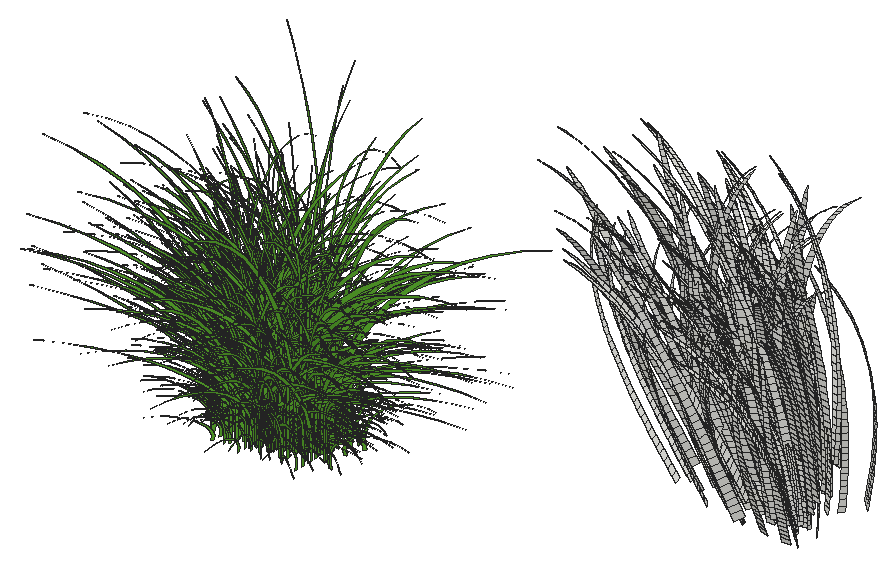
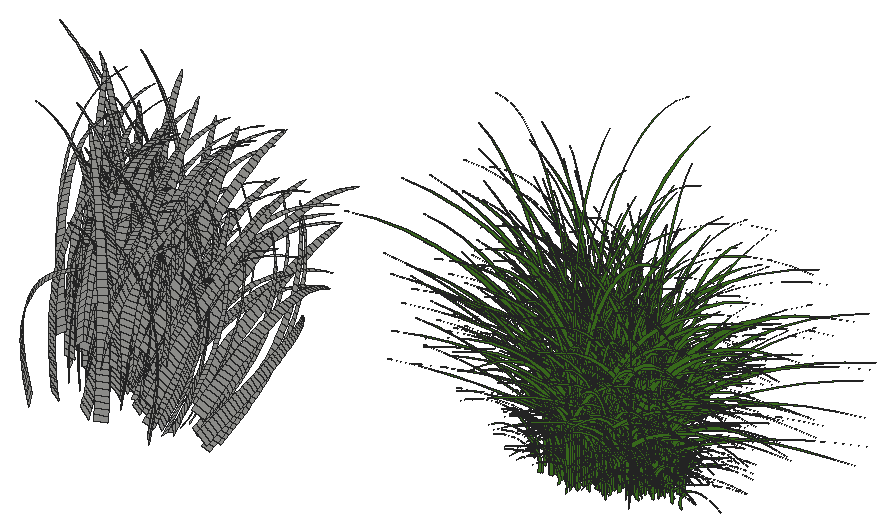
# SketchUp Ruby script. Lengths in inches.
U = 1.inch
M = Sketchup.active_model
def pt(a) = Geom::Point3d.new(a.map { |v| v * U })
def face(e, loops, mat)
  f = e.add_face(loops[0].map { |a| pt(a) })
  loops[1..].each { |l| e.add_face(l.map { |a| pt(a) }).erase! }
  f.material = f.back_material = mat if mat
  f
end
# faces: each face lists its corners as indices into pts; further lists are holes
def faces(e, pts, list, mat = nil) = list.each { |f| face(e, (f[0].is_a?(Array) ? f : [f]).map { |l| l.map { |i| pts[i] } }, mat) }
# xy, xz, yz: faces in a plane at the given z, y or x. An outline is a flat list of corners, or four numbers for a rectangle; further outlines are holes
def ring(l) = l.size == 4 ? [[l[0], l[1]], [l[2], l[1]], [l[2], l[3]], [l[0], l[3]]] : l.each_slice(2).to_a
def flat(e, list, mat, &to3) = list.each { |f| face(e, (f[0].is_a?(Array) ? f : [f]).map { |l| ring(l).map { |u, v| to3.(u, v) } }, mat) }
def xy(e, z, list, mat = nil) = flat(e, list, mat) { |x, y| [x, y, z] }
def xz(e, y, list, mat = nil) = flat(e, list, mat) { |x, z| [x, y, z] }
def yz(e, x, list, mat = nil) = flat(e, list, mat) { |y, z| [x, y, z] }
def lines(e, pts, list) = list.each { |a, b| e.add_line(pt(pts[a]), pt(pts[b])) }
# prism: a flat outline (further loops are holes) pulled along v
def prism(e, loops, v, mat = nil)
  f = face(e, loops, mat); d = Geom::Vector3d.new(v.map { |x| x * U })
  f.pushpull(f.normal.samedirection?(d) ? d.length : -d.length)
end
def box(e, o, s, mat = nil) = prism(e, [[o, [o[0] + s[0], o[1], o[2]], [o[0] + s[0], o[1] + s[1], o[2]], [o[0], o[1] + s[1], o[2]]]], [0, 0, s[2]], mat)
def at(x, y, z, deg = 0) = Geom::Transformation.translation(pt([x, y, z])) * Geom::Transformation.rotation(ORIGIN, Z_AXIS, deg.degrees)
def axes(o, x, y, z) = Geom::Transformation.new([*x, 0, *y, 0, *z, 0, *pt(o).to_a, 1])
def part(name) = M.definitions.add(name)
# library, detail: a bought-in or finely detailed component or shape, given as its bounding box
def library(name, o, s) = part(name).tap { |d| box(d.entities, o, s) }
def detail(e, o, s) = box(e.add_group.entities, o, s)
def put(e, d, t, mat = nil) = e.add_instance(d, t).tap { |i| i.material = mat if mat }
def group(e, t, mat = nil) = e.add_group.tap { |g| g.transformation = t; g.material = mat if mat }.entities
root = M.entities
M.materials.add("[Color_G08]").color = [89, 170, 45]
c1 = part("Miscanthus Gracillimus Blades")
xz(c1.entities,0,[[29.29,0,29.21,4.14,28.62,8.24,27.52,12.24,25.9375,16.07,23.89,19.67,21.41,22.98,18.53,25.97,15.3125,28.57,11.79,30.76,8.03,32.48,4.08,33.73,0,34.48,4.17,33.88,8.22,32.75,12.09,31.1,15.72,28.96,19.03,26.37,21.99,23.37,24.53,20.01,26.61,16.35,28.2,12.45,29.27,8.38,29.8,4.21,29.79,0],[30.59,0,30.59,18.4375,30.42,21.54,29.8,24.59,28.74,27.51,27.27,30.25,25.41,32.74,23.21,34.93,20.7,36.77,17.96,38.23,15.03,39.27,11.98,39.875,8.88,40.02,5.78,39.71,8.9,40.03,12.04,39.89,15.11,39.29,18.07,38.26,20.85,36.81,23.39,34.97,25.64,32.78,27.55,30.29,29.07,27.56,30.19,24.625,30.86,21.5625,31.09,18.4375,31.09,0],[25.43,0,25.6,1.22,25.54,2.45,25.24,3.64,24.72,4.76,24,5.75,23.1,6.59,22.05,7.25,20.9,7.6875,19.69,7.9,18.46,7.875,17.26,7.62,16.125,7.14,17.28,7.63,18.51,7.9,19.77,7.94,21.02,7.74,22.2,7.3125,23.28,6.67,24.23,5.84,25,4.84,25.57,3.72,25.92,2.51,26.04,1.25,25.93,0],[27.07,0,27.07,8.3125,27.03,9.48,26.8,10.63,26.39,11.73,25.8,12.74,25.06,13.64,24.18,14.41,23.18,15.03,22.1,15.48,20.96,15.74,19.79,15.8125,18.63,15.7,17.5,15.39,18.66,15.71,19.85,15.83,21.05,15.77,22.22,15.52,23.34,15.08,24.375,14.47,25.3,13.7,26.09,12.8,26.73,11.78,27.19,10.68,27.48,9.51,27.57,8.3125,27.57,0],[32.33,0,32.33,16.35,32.43,19.17,32.72,21.98,33.19,24.76,33.85,27.5,34.7,30.19,35.73,32.82,36.93,35.37,38.31,37.84,39.84,40.2,41.54,42.46,43.38,44.59,45.37,46.6,43.45,44.56,41.68,42.39,40.04,40.12,38.57,37.74,37.25,35.27,36.09,32.72,35.1,30.1,34.29,27.42,33.66,24.7,33.2,21.93,32.92,19.15,32.83,16.35,32.83,0],
  [33.58,0,33.5625,4.21,34.1,8.38,35.17,12.45,36.76,16.35,38.84,20.01,41.375,23.37,44.33,26.37,47.65,28.96,51.27,31.1,55.14,32.75,59.2,33.88,63.36,34.48,59.29,33.73,55.34,32.48,51.57,30.76,48.05,28.57,44.83,25.97,41.96,22.98,39.48,19.67,37.43,16.07,35.84,12.24,34.75,8.24,34.15,4.14,34.08,0],[36.0625,0,36.0625,8.3125,36.16,9.51,36.44,10.68,36.91,11.78,37.54,12.8,38.34,13.7,39.26,14.47,40.29,15.08,41.41,15.52,42.58,15.77,43.78,15.83,44.98,15.71,46.13,15.39,45,15.7,43.84,15.8125,42.67,15.74,41.53,15.48,40.45,15.03,39.45,14.41,38.57,13.64,37.83,12.74,37.24,11.73,36.83,10.63,36.6,9.48,36.5625,8.3125,36.5625,0],[38.05,0,37.9375,1.25,38.06,2.51,38.41,3.72,38.98,4.84,39.75,5.84,40.7,6.67,41.78,7.3125,42.97,7.74,44.21,7.94,45.47,7.9,46.7,7.63,47.86,7.14,46.72,7.62,45.52,7.875,44.29,7.9,43.08,7.6875,41.93,7.25,40.88,6.59,39.98,5.75,39.26,4.76,38.74,3.64,38.44,2.45,38.38,1.22,38.55,0]],"[Color_G08]")
c2 = part("Grass blade cluster \#1")
put(c2.entities,c1,axes([15.51,50.54,0],[0.60321,-0.79758,0],[0.79758,0.60321,0],[0,0,0.83]))
put(c2.entities,c1,at(0,25.27,0))
c3 = part("Grass blade cluster")
put(c3.entities,c2,axes([30.74,66.43,0],[-0.57215,-0.82015,0],[0.82015,-0.57215,0],[0,0,0.65]))
put(c3.entities,c2,at(0.28,0.71,0))
c4 = part("Grass tuft \#1")
put(c4.entities,c3,at(0,0,0))
put(c4.entities,c3,axes([1.91,58.875,0],[0.17537,-0.9845,0],[0.9845,0.17537,0],[0,0,0.84]))
c5 = part("Grass tuft")
put(c5.entities,c4,at(-0.89,7.45,0))
put(c5.entities,c4,axes([-12.2,31.71,0],[0.80178,-0.59763,0],[0.59763,0.80178,0],[0,0,1.31]))
c6 = part("Ornamental grass clump \#1")
put(c6.entities,c5,axes([-5.64,62.125,0],[0.1788,-0.98389,0],[0.98389,0.1788,0],[0,0,1.27]))
put(c6.entities,c5,at(6.7,0,0))
c7 = part("Ornamental grass clump")
put(c7.entities,c6,at(12.67,21.7,0))
put(c7.entities,c6,axes([-14.56,78.18,0],[0.66352,-1.26381,0],[1.25239,0.65752,0],[0,0,0.9558]))
c8 = part("Miscanthus Gracillimus")
put(c8.entities,c7,axes([-6.55,172.36,0],[-0.09268,-1.60733,0],[1.41765,-0.08174,0],[0,0,1.1742]))
put(c8.entities,c7,at(11.73,20.84,0))
c9 = part("Misc Gracillimus")
put(c9.entities,c8,at(-70.11,-74.01,2.38))
c10 = part("fur_instance\#8")
p = [[-0.25,1.49,0.03],[0.25,-1.49,-0.03],[0.44,-1.47,1.51],[-0.05,1.47,1.57],[0.65,-1.44,3.05],[0.16,1.45,3.11],
  [0.86,-1.42,4.59],[0.38,1.44,4.65],[1.1,-1.39,6.13],[0.62,1.43,6.18],[1.34,-1.35,7.66],[0.875,1.42,7.72],
  [1.6,-1.32,9.19],[1.14,1.41,9.25],[1.88,-1.28,10.72],[1.43,1.41,10.78],[2.18,-1.24,12.25],[1.73,1.41,12.3],
  [2.49,-1.19,13.77],[2.05,1.41,13.82],[2.83,-1.15,15.29],[2.4,1.41,15.34],[3.18,-1.09,16.8],[2.76,1.42,16.85],
  [3.56,-1.03,18.31],[3.14,1.43,18.35],[3.96,-0.97,19.81],[3.55,1.44,19.85],[4.38,-0.91,21.3],[3.99,1.46,21.35],
  [4.84,-0.83,22.78],[4.45,1.48,22.83],[5.32,-0.76,24.26],[4.93,1.51,24.31],[5.82,-0.67,25.73],[5.45,1.54,25.77],
  [6.36,-0.59,27.18],[6,1.57,27.23],[6.93,-0.49,28.625],[6.58,1.61,28.67],[7.54,-0.39,30.05],[7.19,1.66,30.1],
  [8.18,-0.28,31.47],[7.84,1.71,31.51],[8.85,-0.16,32.86],[8.53,1.77,32.9],[9.57,-0.04,34.24],[9.25,1.83,34.27],
  [10.32,0.09,35.59],[10.02,1.9,35.625],[11.12,0.23,36.92],[10.82,1.97,36.95],[11.95,0.38,38.22],[11.67,2.06,38.25],
  [12.84,0.54,39.49],[12.57,2.14,39.52],[13.76,0.71,40.73],[13.51,2.24,40.76],[14.73,0.89,41.93],[14.49,2.34,41.95],
  [15.75,1.08,43.09],[15.52,2.45,43.11],[16.82,1.28,44.2],[16.6,2.5625,44.23],[17.93,1.5,45.27],[17.73,2.68,45.29],
  [19.08,1.73,46.28],[18.9,2.81,46.3],[20.29,1.97,47.24],[20.125,2.93,47.26],[21.53,2.22,48.13],[21.39,3.0625,48.15],
  [22.82,2.5,48.96],[22.7,3.1875,48.98],[24.14,2.8125,49.72],[24.06,3.3,49.73],[25.48,3.27,50.41]]
faces(c10.entities,p,[[0,1,2,3],[3,2,4,5],[5,4,6,7],[7,6,8,9],[9,8,10,11],[11,10,12,13],[13,12,14,15],[15,14,16,17],
  [17,16,18,19],[19,18,20,21],[21,20,22,23],[23,22,24,25],[25,24,26,27],[27,26,28,29],[29,28,30,31],[31,30,32,33],
  [33,32,34,35],[35,34,36,37],[37,36,38,39],[39,38,40,41],[41,40,42,43],[43,42,44,45],[45,44,46,47],[47,46,48,49],
  [49,48,50,51],[51,50,52,53],[53,52,54,55],[55,54,56,57],[57,56,58,59],[59,58,60,61],[61,60,62,63],[63,62,64,65],
  [65,64,66,67],[67,66,68,69],[69,68,70,71],[71,70,72,73],[73,72,74,75],[75,74,76]])
put(root,c9,axes([127.3,24.12,14.73],[0.40613,0,0],[0,0.23,0],[0,0,0.45908]))
put(root,c10,axes([161.89,46.04,18.83],[-0.11569,0.14649,-0.11362],[-0.49612,-0.01353,-0.24569],[-0.28238,-0.00989,0.50725]))
put(root,c10,axes([161.84,45.54,15.92],[0.13882,0.1225,0.02997],[-0.38832,0.05902,-0.33485],[-0.34424,0.00121,0.41007]))
put(root,c10,axes([164.85,44.78,21.47],[-0.38731,-0.08952,-0.1497],[0.42326,-0.11791,0.09629],[-0.18899,-0.03826,0.56909]))
put(root,c10,axes([167.375,46.33,21.8],[-0.5712,-0.00621,-0.12571],[0.08241,-0.15116,0.10787],[-0.15761,-0.00674,0.56684]))
put(root,c10,axes([161.46,45.36,14.86],[0.25376,-0.11142,0.26435],[0.3129,0.07232,0.1949],[-0.33629,0.00118,0.40061]))
put(root,c10,axes([164.68,43.97,18.74],[-0.09562,-0.12227,-0.11226],[0.47205,-0.05859,0.23599],[-0.27058,-0.03426,0.47864]))
put(root,c10,axes([161.26,43.68,14.85],[0.37582,-0.08407,0.27007],[0.14827,0.09994,0.19932],[-0.3433,-0.03091,0.40153]))
put(root,c10,axes([167.84,43.74,19.98],[-0.45134,-0.04336,-0.16335],[0.26487,-0.12485,0.01208],[-0.16324,-0.04231,0.51575]))
put(root,c10,axes([166.53,47.59,18.875],[-0.27902,-0.12125,0.0786],[0.46466,-0.07901,0.25002],[-0.20176,0.02209,0.50718]))
put(root,c10,axes([169.09,42.55,17.125],[-0.34603,0.08867,-0.06121],[-0.25159,-0.06276,-0.21848],[-0.20018,-0.04995,0.40733]))
put(root,c10,axes([163.27,43.46,15.76],[0.37143,-0.07872,0.26996],[0.13229,0.10024,0.18556],[-0.33504,-0.03016,0.39186]))
put(root,c10,axes([164.23,43.5,14.97],[0.28927,0.04096,0.28152],[-0.23066,0.11236,-0.1234],[-0.31438,-0.0283,0.3677]))
put(root,c10,axes([170.18,42.21,17.68],[-0.42495,0.07188,-0.0749],[-0.17281,-0.08134,-0.22626],[-0.18095,-0.06165,0.42446]))
put(root,c10,axes([170.17,44.48,19],[-0.46693,0.04407,-0.14017],[-0.11268,-0.11869,0.01707],[-0.14651,-0.01142,0.47518]))
put(root,c10,axes([169.15,43.8125,16.33],[-0.24594,-0.08141,-0.04983],[0.3096,-0.07753,0.19842],[-0.20231,0.00171,0.38778]))
put(root,c10,axes([169.08,45.1,22.68],[-0.21709,-0.12668,-0.07521],[0.52524,-0.07803,0.15682],[-0.18992,-0.02954,0.56536]))
put(root,c10,axes([171.66,41.45,17.58],[-0.54111,0.06042,0.07587],[-0.19981,-0.07219,-0.37016],[-0.0944,-0.11415,0.43604]))
put(root,c10,axes([165.41,44.12,15.41],[0.35881,-0.03428,0.29675],[0.0665,0.11534,-0.02105],[-0.30461,0.00107,0.36287]))
put(root,c10,axes([171.71,43.03,20.65],[-0.51581,-0.0175,-0.13293],[0.18056,-0.12516,-0.10858],[-0.10807,-0.06258,0.52244]))
put(root,c10,axes([169.72,42.74,18.6],[-0.0707,0.11438,0.11912],[-0.45161,0.01974,-0.21113],[-0.21388,-0.05337,0.43522]))
put(root,c10,axes([167.97,46.0625,15.54],[0.03855,-0.11777,0.25787],[0.43699,0.01768,0.16073],[-0.22604,0.03772,0.38076]))
put(root,c10,axes([170.29,42.21,17.16],[-0.17604,0.10245,0.09767],[-0.39708,-0.00819,-0.20343],[-0.17133,-0.05837,0.40189]))
put(root,c10,axes([171.36,45.2,23.02],[-0.45394,0.1084,-0.0434],[-0.38463,-0.10138,-0.03875],[-0.07351,-0.03167,0.58893]))
put(root,c10,axes([171.03,43.33,17.5],[-0.33805,-0.05461,-0.08887],[0.25639,-0.0976,0.0914],[-0.13824,-0.01588,0.42164]))
put(root,c10,axes([171.04,42.7,17.68],[-0.30117,0.09238,-0.04137],[-0.31304,-0.05917,-0.12952],[-0.1355,-0.03512,0.42811]))
put(root,c10,axes([168.51,44.0625,21.67],[-0.03124,0.13752,0.09977],[-0.56507,0.02087,-0.1473],[-0.1601,-0.0531,0.55264]))
put(root,c10,axes([171.375,45.45,22.85],[-0.45617,0.10631,-0.04963],[-0.37724,-0.10346,-0.0161],[-0.06368,-0.02656,0.58538]))
put(root,c10,axes([170.98,40.94,15.21],[-0.3561,0.08998,0.2615],[-0.45823,-0.02957,-0.27591],[-0.09498,-0.11484,0.43869]))
put(root,c10,axes([171.01,44.45,21.5625],[-0.4634,-0.06206,-0.05309],[0.30711,-0.12341,0.02068],[-0.07005,-0.0322,0.55017]))
put(root,c10,axes([172.18,44.375,22.7],[-0.5539,-0.03134,-0.06208],[0.19807,-0.14029,-0.02574],[-0.06505,-0.0422,0.58034]))
put(root,c10,axes([166.72,44.78,18.39],[0.29385,0.08784,0.11548],[-0.34758,0.09777,-0.2125],[-0.25229,-0.00884,0.4532]))
put(root,c10,axes([166.67,44.3,14.51],[0.29692,-0.06479,0.27774],[0.20048,0.09221,0.0267],[-0.26969,0.01357,0.34365]))
put(root,c10,axes([165.39,45.5,15.54],[0.41573,0.01969,0.20437],[-0.05133,0.12132,-0.2303],[-0.26854,0.02752,0.38268]))
put(root,c10,axes([169.29,44.83,18.13],[0.01538,0.12452,-0.12889],[-0.45208,0.01116,-0.18619],[-0.2031,0.01115,0.43393]))
put(root,c10,axes([166.09,42.1,14.68],[0.4031,-0.04126,0.25346],[-0.04162,0.10161,0.18282],[-0.27306,-0.05722,0.36744]))
put(root,c10,axes([166.92,45.77,15.81],[0.34512,0.07258,0.07648],[-0.23439,0.09857,-0.29696],[-0.26745,0.02741,0.38113]))
put(root,c10,axes([170.17,43.64,14.86],[-0.04139,-0.09921,0.1408],[0.33679,-0.00837,0.20587],[-0.21754,0.02229,0.31]))
put(root,c10,axes([171.3125,41.54,17.35],[-0.27848,0.1037,0.16149],[-0.44453,-0.029,-0.20606],[-0.11622,-0.08309,0.46124]))
put(root,c10,axes([166.42,45.57,14.84],[0.36852,-0.04563,0.28569],[0.16966,0.10995,-0.08547],[-0.26008,0.02666,0.37063]))
put(root,c10,axes([171.5,43.61,14.88],[-0.20225,-0.07964,0.07154],[0.28157,-0.05014,0.22923],[-0.17863,0.02981,0.3009]))
put(root,c10,axes([173.4,44.29,22.76],[-0.55642,0.06257,-0.01207],[-0.1944,-0.1278,-0.0692],[-0.04939,-0.04658,0.57961]))
put(root,c10,axes([168.125,42.74,14.57],[0.31297,-0.02783,0.26111],[0.01775,0.10078,0.01553],[-0.27274,-0.01149,0.31594]))
put(root,c10,axes([172.91,43.47,16.54],[-0.31878,-0.05388,-0.02498],[0.21365,-0.08716,0.18387],[-0.14285,0.01564,0.3591]))
put(root,c10,axes([173.13,49.42,16.5],[-0.47347,-0.07401,0.17022],[0.33824,-0.11173,0.31464],[-0.07498,0.064,0.45544]))
put(root,c10,axes([172.2,43.33,21.07],[-0.25642,0.12058,0.08666],[-0.4804,-0.03631,-0.14745],[-0.10769,-0.06235,0.52058]))
put(root,c10,axes([169.71,42.33,15.98],[0.06935,-0.10181,-0.05617],[0.37358,-0.01131,0.19685],[-0.19972,-0.03626,0.371]))
put(root,c10,axes([168.31,43.01,16.91],[0.28717,0.05906,0.18907],[-0.28878,0.09826,-0.11438],[-0.2288,-0.02897,0.40472]))
put(root,c10,axes([173.67,42.95,17.48],[-0.35379,-0.03909,-0.07768],[0.19159,-0.09858,0.08919],[-0.12272,-0.00957,0.39802]))
put(root,c10,axes([173.29,42.43,16.625],[-0.28182,0.07508,-0.08197],[-0.24497,-0.06261,-0.07961],[-0.12478,-0.01941,0.37146]))
put(root,c10,axes([169.82,43.23,17.05],[0.24853,0.07082,0.13756],[-0.2987,0.08669,-0.15855],[-0.22219,-0.01756,0.38881]))
put(root,c10,axes([171.39,46.29,21.64],[-0.09016,0.14644,-0.14213],[-0.56355,-0.01096,-0.06546],[-0.10497,0.00344,0.55103]))
put(root,c10,axes([173.06,41.56,16.45],[-0.17655,0.0893,0.11813],[-0.36927,-0.01088,-0.17139],[-0.12725,-0.06066,0.36837]))
put(root,c10,axes([166.32,47.12,18.26],[0.49159,0.04485,0.09037],[-0.18613,0.133,-0.23756],[-0.19567,0.02142,0.49187]))
put(root,c10,axes([174.73,41.97,19.27],[-0.54515,0.00019,-0.04346],[0.08112,-0.10399,-0.26579],[-0.02004,-0.09315,0.47314]))
put(root,c10,axes([173.63,43.34,20.02],[-0.38338,-0.06825,-0.0577],[0.32906,-0.10289,-0.00157],[-0.05587,-0.03625,0.49844]))
put(root,c10,axes([166.3125,48.24,15.5],[0.51684,0.0215,0.1164],[-0.05837,0.1295,-0.32132],[-0.20042,0.05174,0.43122]))
put(root,c10,axes([174.5625,42.51,18.33],[-0.42742,0.04491,-0.01878],[-0.13382,-0.09906,-0.04894],[-0.04414,-0.0339,0.44116]))
put(root,c10,axes([174,45.72,20.46],[-0.3694,0.10768,-0.12097],[-0.39548,-0.08499,0.0781],[-0.04054,0.00726,0.51598]))
put(root,c10,axes([171.56,45.57,21.32],[-0.06999,-0.1388,0.09222],[0.54267,-0.03086,0.12251],[-0.12696,-0.00089,0.53285]))
put(root,c10,axes([170.37,42.1,17.375],[0.20583,0.07337,0.22786],[-0.40086,0.07736,-0.05373],[-0.17774,-0.06055,0.41693]))
put(root,c10,axes([174.82,44.43,21.88],[-0.44292,-0.07247,-0.01487],[0.33674,-0.11929,0.04408],[-0.05271,-0.02311,0.54972]))
put(root,c10,axes([172.51,43.86,17.97],[-0.1635,-0.10272,0.04784],[0.41176,-0.05199,0.11457],[-0.1028,-0.00072,0.43144]))
put(root,c10,axes([171.69,42.21,19.13],[-0.00018,0.10449,0.24912],[-0.53072,0.0308,-0.09002],[-0.11758,-0.08407,0.46666]))
put(root,c10,axes([175.04,43.02,17.35],[-0.378,-0.02814,-0.02544],[0.14155,-0.09997,0.10771],[-0.07424,0.00243,0.38971]))
put(root,c10,axes([173.23,43.25,16.97],[-0.18086,-0.08793,0.01093],[0.35575,-0.05669,0.11402],[-0.10899,-0.00466,0.39198]))
put(root,c10,axes([168.98,42.29,16.65],[0.36206,-0.08311,0.07727],[0.22303,0.06894,0.21187],[-0.19897,-0.04965,0.40487]))
put(root,c10,axes([175.14,46.77,16.36],[-0.50255,-0.00379,0.04989],[0.06422,-0.11586,0.30455],[-0.00175,0.05488,0.39355]))
put(root,c10,axes([171.48,41.82,17.45],[0.11839,0.08702,0.23179],[-0.45761,0.05675,-0.0637],[-0.14695,-0.07005,0.4254]))
put(root,c10,axes([174.02,45.53,22.4],[-0.30008,0.13108,-0.04422],[-0.4957,-0.06287,0.00183],[-0.03589,-0.02154,0.57138]))
put(root,c10,axes([175.21,43.53,18.26],[-0.43075,0.03793,-0.02322],[-0.10996,-0.10489,0.02478],[-0.02753,-0.01653,0.43837]))
put(root,c10,axes([172.71,43.81,20.7],[-0.12159,0.12941,0.00902],[-0.51234,-0.01443,-0.05556],[-0.06562,-0.03301,0.52078]))
put(root,c10,axes([172.93,42.79,19.19],[-0.10684,-0.10313,-0.13113],[0.46435,-0.04764,0.07264],[-0.11632,-0.0501,0.46037]))
put(root,c10,axes([171.8125,42.74,18.23],[0.03094,-0.11145,-0.05259],[0.44379,-0.01421,0.12893],[-0.13876,-0.03596,0.43843]))
put(root,c10,axes([170.77,41.62,14.42],[0.30819,-0.01996,0.21867],[-0.08034,0.08385,0.11184],[-0.2146,-0.04497,0.28878]))
put(root,c10,axes([174.24,41.73,17.72],[-0.33936,-0.05842,-0.11874],[0.32052,-0.08468,-0.0844],[-0.04225,-0.05911,0.43914]))
put(root,c10,axes([166.82,44.84,21.55],[0.55538,-0.04347,0.16105],[0.07,0.13775,0.06498],[-0.1844,-0.03733,0.55525]))
put(root,c10,axes([175.91,42.67,20.23],[-0.51823,-0.01807,-0.01549],[0.12857,-0.11474,-0.16499],[0.01257,-0.06919,0.5005]))
put(root,c10,axes([176.18,46.5,21.87],[-0.53194,0.07351,-0.03034],[-0.24436,-0.12866,0.15206],[0.02284,0.00582,0.55711]))
put(root,c10,axes([173.2,43.58,19.65],[-0.10827,0.12148,-0.00042],[-0.4794,-0.01253,-0.05037],[-0.06193,-0.02846,0.48638]))
put(root,c10,axes([176.08,45.47,17.01],[-0.47413,0.01058,0.00606],[-0.00201,-0.1159,0.21118],[-0.00511,0.02935,0.41767]))
put(root,c10,axes([175.33,45.54,22.07],[-0.35953,0.11919,-0.03229],[-0.44475,-0.07957,0.02653],[-0.0137,-0.02083,0.56315]))
put(root,c10,axes([167.76,43.45,21.03],[0.48701,0.04757,0.174],[-0.30593,0.1286,0.04964],[-0.14041,-0.06048,0.55568]))
put(root,c10,axes([168.58,44.0625,19.04],[0.45655,0.02353,0.14229],[-0.16482,0.12487,-0.04265],[-0.1622,-0.02523,0.48286]))
put(root,c10,axes([171.72,43.33,15.77],[0.19405,-0.08782,0.16981],[0.30748,0.04885,0.06553],[-0.16325,0.00896,0.34879]))
put(root,c10,axes([168.82,46.38,18.31],[0.49985,0.00301,0.14964],[-0.02964,0.13367,-0.19035],[-0.18639,0.02041,0.46856]))
put(root,c10,axes([170.82,41.34,14.85],[0.32877,0.00795,0.24484],[-0.22697,0.08276,0.1343],[-0.16825,-0.07161,0.32423]))
put(root,c10,axes([175.875,41.83,16.48],[-0.33843,0.04553,-0.01108],[-0.1473,-0.07721,-0.04176],[-0.03638,-0.02793,0.36355]))
put(root,c10,axes([176.27,44.27,18.79],[-0.41033,0.06923,-0.06032],[-0.23945,-0.09817,0.11027],[-0.00841,0.00619,0.45189]))
put(root,c10,axes([174.74,41.87,16.42],[-0.0905,0.08851,0.04381],[-0.349,-0.00424,-0.10453],[-0.10199,-0.03383,0.35208]))
put(root,c10,axes([175.46,42.67,18.45],[-0.3213,-0.06561,-0.05115],[0.31218,-0.08598,-0.01531],[-0.03754,-0.0354,0.44054]))
put(root,c10,axes([172.41,44.84,19.38],[0.08835,0.12369,-0.09809],[-0.4898,0.03322,-0.09487],[-0.09155,0.003,0.48054]))
put(root,c10,axes([176.61,42.4,18.56],[-0.43764,0.04296,0.02293],[-0.13889,-0.10078,-0.05047],[-0.0046,-0.03883,0.44986]))
put(root,c10,axes([174.37,43.59,21.06],[-0.16558,0.12699,0.05128],[-0.5131,-0.0254,-0.04],[-0.03606,-0.04403,0.52943]))
put(root,c10,axes([174.625,42.89,18.2],[-0.21313,-0.08851,-0.02181],[0.38204,-0.06383,0.0368],[-0.05405,-0.02329,0.43302]))
put(root,c10,axes([172.74,42.17,15.75],[0.21366,-0.07915,0.11274],[0.23837,0.04733,0.13112],[-0.18304,-0.01446,0.32031]))
put(root,c10,axes([175.76,43.25,15.53],[-0.30076,-0.04712,0.07311],[0.21058,-0.07732,0.14762],[-0.03812,0.02306,0.32501]))
put(root,c10,axes([170.98,49.66,16.41],[0.13416,-0.13299,0.35981],[0.57303,0.02622,-0.03812],[-0.07584,0.06473,0.46065]))
put(root,c10,axes([171.11,41.375,15.08],[0.36016,-0.00742,0.21279],[-0.15994,0.08168,0.17492],[-0.16596,-0.07064,0.31982]))
put(root,c10,axes([174.58,42.38,16.63],[0.00161,0.09513,-0.03701],[-0.36368,0.01178,-0.1003],[-0.11093,-0.00865,0.35978]))
put(root,c10,axes([169.46,44.52,19.93],[0.49874,-0.00013,0.14505],[-0.06914,0.13272,-0.04302],[-0.16406,-0.01885,0.50038]))
put(root,c10,axes([174.38,44.55,17.86],[-0.13345,-0.10841,0.09578],[0.43742,-0.04305,0.07746],[-0.05987,0.00506,0.43831]))
put(root,c10,axes([176.63,42.12,18.27],[-0.43123,-0.02453,-0.02633],[0.15077,-0.0963,-0.13931],[0.01076,-0.0592,0.42821]))
put(root,c10,axes([176.64,41.89,16.83],[-0.36718,0.0373,0.01282],[-0.1193,-0.08429,-0.04508],[-0.0113,-0.03262,0.37838]))
put(root,c10,axes([177.61,40.99,16.42],[-0.58089,-0.00691,0.01192],[0.06233,-0.08859,-0.37865],[0.05076,-0.11892,0.43771]))
put(root,c10,axes([176.03,42.23,17.85],[-0.25951,0.08816,0.03471],[-0.34222,-0.05282,-0.03889],[-0.02082,-0.03587,0.42124]))
put(root,c10,axes([174.29,42.03,19.67],[-0.09978,0.10955,0.27884],[-0.57213,-0.00253,-0.05277],[-0.02112,-0.09816,0.49856]))
put(root,c10,axes([174.36,44.22,20.4],[-0.05866,0.12941,-0.03315],[-0.51241,-0.00175,-0.02422],[-0.04091,-0.02008,0.50906]))
put(root,c10,axes([173.59,42.7,16.875],[0.16807,0.08479,0.01084],[-0.34402,0.05473,-0.11203],[-0.11678,-0.00911,0.37877]))
put(root,c10,axes([177.89,43.56,19.08],[-0.46606,0.03056,0.02824],[-0.08561,-0.11409,0.02579],[0.02128,-0.02161,0.46667]))
put(root,c10,axes([175.11,44.1,19.19],[-0.16336,-0.11028,0.11018],[0.45015,-0.05074,0.06399],[-0.03587,0.00642,0.45659]))
put(root,c10,axes([176.53,42.77,16.61],[-0.27897,0.07131,-0.06646],[-0.25904,-0.06465,0.07567],[-0.00674,0.00496,0.3621]))
put(root,c10,axes([175.35,41.21,16.65],[-0.14342,0.08904,0.22161],[-0.45562,-0.01395,-0.07327],[-0.01737,-0.08073,0.41005]))
put(root,c10,axes([172.18,46.64,20.8125],[0.23264,0.12597,-0.10506],[-0.51463,0.06987,-0.11002],[-0.07393,0.00625,0.54129]))
put(root,c10,axes([178.23,40.78,15.3],[-0.52353,-0.00648,0.00968],[0.05783,-0.07985,-0.3414],[0.04576,-0.10721,0.39462]))
put(root,c10,axes([174.79,41.77,18.16],[0.0088,0.09179,0.23634],[-0.48628,0.02291,-0.03823],[-0.06294,-0.08038,0.42075]))
put(root,c10,axes([175.03,41.93,16.33],[-0.10781,-0.08139,-0.03075],[0.34692,-0.03681,0.02599],[-0.04337,-0.02447,0.35891]))
put(root,c10,axes([172.83,42.66,18.03],[0.30249,0.06001,0.12673],[-0.30247,0.08983,-0.04319],[-0.13343,-0.03458,0.42158]))
put(root,c10,axes([175.1875,41.71,17.66],[-0.04888,0.1009,0.13652],[-0.45572,0.00466,-0.04266],[-0.04148,-0.05804,0.43118]))
put(root,c10,axes([176.73,42.17,17.97],[-0.30018,-0.06861,-0.03377],[0.31765,-0.07853,-0.04055],[-0.00438,-0.03696,0.4282]))
put(root,c10,axes([177.125,42.77,16.85],[-0.32765,0.05974,-0.03347],[-0.20786,-0.07797,0.09718],[0.01514,0.00386,0.36928]))
put(root,c10,axes([175.54,42.25,18.4],[-0.06636,0.10018,0.13362],[-0.44971,0.00065,-0.04765],[-0.04114,-0.05756,0.42765]))
put(root,c10,axes([170.79,43.52,20.57],[0.50715,0.00443,0.15053],[-0.1243,0.12826,0.06546],[-0.14771,-0.04899,0.5099]))
put(root,c10,axes([171.9375,46.28,17.98],[0.34405,0.08969,-0.10867],[-0.37288,0.09039,-0.20447],[-0.09963,0.03029,0.45484]))
put(root,c10,axes([177.7,41.74,18.59],[-0.36447,0.07896,0.21772],[-0.39598,-0.06356,-0.1473],[0.03027,-0.09135,0.46262]))
put(root,c10,axes([178.44,45.32,16.59],[-0.4647,0.01323,0.04334],[-0.00327,-0.11424,0.20324],[0.03787,0.02653,0.41066]))
put(root,c10,axes([177.5625,41.24,16.35],[-0.37581,-0.02932,-0.06012],[0.18095,-0.07288,-0.19466],[0.02346,-0.0708,0.35854]))
put(root,c10,axes([177.17,41.8,17.38],[-0.31257,-0.05643,-0.07382],[0.28766,-0.07317,-0.10923],[0.01,-0.05505,0.39818]))
put(root,c10,axes([175.18,42.19,18.17],[-0.01001,-0.09792,-0.13074],[0.44408,-0.02005,0.04748],[-0.0648,-0.05406,0.42072]))
put(root,c10,axes([175.27,42.65,16.95],[-0.01158,0.09749,-0.01907],[-0.38954,0.00726,-0.02642],[-0.03692,-0.01619,0.38504]))
put(root,c10,axes([172.88,44.19,15.07],[0.37509,-0.00503,0.13269],[0.03952,0.09506,-0.20931],[-0.14533,0.03752,0.3127]))
put(root,c10,axes([177.54,43.61,15.21],[-0.35156,-0.02343,0.09214],[0.13344,-0.09006,0.14067],[0.03064,0.02147,0.3323]))
put(root,c10,axes([178.42,44.54,19.37],[-0.48282,0.03787,0.05564],[-0.10728,-0.12068,0.12175],[0.07138,-0.00192,0.47478]))
put(root,c10,axes([177.45,43.41,15.79],[-0.3432,-0.03128,0.10487],[0.16444,-0.08883,0.13403],[0.03101,0.02173,0.3363]))
put(root,c10,axes([174.09,40.89,14.77],[0.24402,0.02996,0.24172],[-0.30035,0.06388,0.09644],[-0.11278,-0.07371,0.30098]))
put(root,c10,axes([175.19,42.75,17.6],[-0.01904,-0.10265,0.01189],[0.41404,-0.01593,0.03454],[-0.04459,-0.0186,0.40988]))
put(root,c10,axes([170.86,45.4,19.31],[0.49255,-0.04177,0.1216],[0.11668,0.12473,-0.07304],[-0.11745,-0.00082,0.49294]))
put(root,c10,axes([177.83,41.18,15.8],[-0.32988,0.03943,0.08],[-0.16177,-0.07038,-0.08094],[0.02899,-0.04686,0.34555]))
put(root,c10,axes([176.4375,41.98,16.98],[-0.10109,0.09263,0.04271],[-0.37836,-0.0142,-0.02086],[-0.01898,-0.0327,0.38411]))
put(root,c10,axes([177.9375,41.53,17.2],[-0.32936,0.06808,0.11834],[-0.29249,-0.0687,-0.06791],[0.03475,-0.05618,0.41428]))
put(root,c10,axes([173.2,42.66,17.73],[0.37819,0.02332,0.12618],[-0.16081,0.10345,-0.01829],[-0.13537,-0.0274,0.40764]))
put(root,c10,axes([178.53,43.06,19.57],[-0.40842,-0.06021,0.01761],[0.27772,-0.10386,-0.0502],[0.03133,-0.03581,0.48562]))
put(root,c10,axes([179.55,49.79,15.875],[-0.57806,0.05108,-0.01731],[-0.12104,-0.11425,0.44744],[0.09241,0.08506,0.38432]))
put(root,c10,axes([176.875,43.49,16.64],[-0.19202,-0.08498,0.095],[0.35389,-0.05606,0.04819],[-0.00713,0.00524,0.38297]))
put(root,c10,axes([173.51,43.82,18.01],[0.27598,-0.0948,0.12215],[0.34126,0.0634,0.01439],[-0.10184,-0.00071,0.42741]))
put(root,c10,axes([172.29,43.61,17.63],[0.42778,-0.01339,0.10479],[0.00746,0.11136,-0.06402],[-0.11685,-0.005,0.42023]))
put(root,c10,axes([178.38,47.48,15.7],[-0.43423,-0.05189,0.22625],[0.28979,-0.11034,0.22684],[0.06324,0.05342,0.40843]))
put(root,c10,axes([177.97,41.66,16.64],[-0.34199,0.0411,0.09804],[-0.17435,-0.07537,-0.06688],[0.05023,-0.04727,0.36326]))
put(root,c10,axes([178.83,43.1,20.66],[-0.51474,-0.03184,0.06575],[0.14327,-0.11828,-0.15109],[0.0949,-0.06218,0.50971]))
put(root,c10,axes([178.85,45.89,21.8],[-0.45361,0.09931,-0.00173],[-0.35091,-0.10792,0.15521],[0.08277,-0.00223,0.55052]))
put(root,c10,axes([177.18,42.79,19.83],[-0.15441,0.11801,0.06042],[-0.4822,-0.02651,-0.00202],[0.00435,-0.04241,0.49616]))
put(root,c10,axes([173.54,43.65,15.58],[0.34239,0.03726,0.01765],[-0.15602,0.08967,-0.17532],[-0.10788,0.01972,0.34387]))
put(root,c10,axes([177.46,43.9,17.51],[-0.25273,-0.08422,0.10734],[0.35641,-0.07169,0.04327],[0.01705,0.00435,0.41582]))
put(root,c10,axes([173.34,42.39,17.09],[0.38587,-0.03244,0.1112],[0.05744,0.0953,0.04779],[-0.12851,-0.02601,0.38698]))
put(root,c10,axes([178.51,43.51,14.9],[-0.36631,0.00606,0.06098],[0.02871,-0.0856,0.21709],[0.04451,0.0376,0.28747]))
put(root,c10,axes([174.26,45.09,16.65],[0.12621,-0.10931,0.20195],[0.43609,0.02424,-0.02656],[-0.04713,0.02851,0.40188]))
put(root,c10,axes([173.81,42.28,16.49],[0.3508,0.01,0.1088],[-0.09536,0.09464,-0.02321],[-0.12148,-0.01889,0.36163]))
put(root,c10,axes([175.89,41.27,16.22],[0.06624,0.0707,0.19388],[-0.38826,0.02952,-0.00183],[-0.05097,-0.06509,0.34074]))
put(root,c10,axes([174.55,41.36,15.83],[0.21052,0.05846,0.11488],[-0.3,0.06136,0.00722],[-0.07248,-0.04197,0.35036]))
put(root,c10,axes([176.25,41.53,16.26],[0.01274,0.07928,0.11279],[-0.36595,0.01506,-0.01834],[-0.03314,-0.04637,0.34447]))
put(root,c10,axes([172.26,42.69,19.03],[0.47736,-0.00825,0.11552],[-0.0647,0.11455,0.0981],[-0.11761,-0.05065,0.46544]))
put(root,c10,axes([175.47,44.12,18.02],[0.01936,-0.11455,0.11924],[0.45185,-0.00462,0.01622],[-0.03388,0.00606,0.43122]))
put(root,c10,axes([179,44.32,17.29],[-0.42384,0.04557,0.02145],[-0.12975,-0.1021,0.19976],[0.07609,0.02143,0.39589]))
put(root,c10,axes([174.14,41.97,16.92],[0.31358,0.03997,0.1214],[-0.23702,0.08477,0.02354],[-0.09596,-0.04133,0.37979]))
put(root,c10,axes([179.35,45.38,22.26],[-0.55439,0.04219,0.1189],[-0.1271,-0.14066,0.10699],[0.12892,-0.0151,0.55302]))
put(root,c10,axes([173.08,43.76,19.42],[0.28313,-0.10582,0.03214],[0.39385,0.05937,0.03161],[-0.0569,-0.02368,0.47998]))
put(root,c10,axes([175.92,45.71,20.85],[-0.04433,-0.13714,0.14531],[0.54821,-0.02307,0.0077],[-0.00974,0.00716,0.52315]))
put(root,c10,axes([178.41,42.53,17.88],[-0.29839,-0.07028,0.01347],[0.30944,-0.0781,-0.04239],[0.0299,-0.02932,0.42303]))
put(root,c10,axes([174.77,42.68,20.86],[0.0693,-0.12441,-0.17586],[0.56699,0.00008,0.02563],[-0.01912,-0.07384,0.53545]))
put(root,c10,axes([172.53,47.04,22.28],[0.44782,0.09145,-0.05384],[-0.39648,0.12211,-0.15184],[-0.0783,0.00662,0.57325]))
put(root,c10,axes([178.11,41.86,16.48],[-0.19649,0.07966,0.03715],[-0.31445,-0.04216,0.01466],[0.02352,-0.02689,0.36458]))
put(root,c10,axes([177.15,43.92,17.83],[-0.09892,0.11156,-0.10569],[-0.43367,-0.01525,0.05209],[0.01735,0.00442,0.42332]))
put(root,c10,axes([178.46,43.3,18.76],[-0.27782,-0.08651,0.03255],[0.37049,-0.07598,-0.02201],[0.0263,-0.02299,0.45617]))
put(root,c10,axes([178.625,43.45,21.49],[-0.43152,-0.0789,0.00058],[0.34787,-0.0996,-0.17093],[0.09845,-0.06451,0.52876]))
put(root,c10,axes([177.49,42.35,17.25],[-0.18439,-0.08403,0.01453],[0.35469,-0.05174,-0.03473],[0.02823,-0.02351,0.39379]))
put(root,c10,axes([177.47,42.61,17.66],[-0.18001,-0.08959,0.01998],[0.37595,-0.05144,-0.03146],[0.02729,-0.02255,0.41065]))
put(root,c10,axes([174.06,42.72,18.19],[0.3037,0.06869,0.04741],[-0.31921,0.08377,-0.01172],[-0.0526,-0.02968,0.43528]))
put(root,c10,axes([177.59,42.3,16.85],[-0.165,-0.08272,0.02284],[0.34646,-0.04755,-0.02321],[0.02179,-0.01905,0.37802]))
put(root,c10,axes([171.99,42.93,20.59],[0.5234,0.01758,0.11027],[-0.1743,0.12288,0.13297],[-0.08048,-0.06713,0.52251]))
put(root,c10,axes([178.59,44.99,18.78],[-0.28571,-0.09566,0.12989],[0.4032,-0.08143,0.02314],[0.04626,0.00211,0.47184]))
put(root,c10,axes([176.89,43.7,19.14],[-0.07524,-0.11534,0.03315],[0.46935,-0.02879,-0.01273],[0.00642,-0.01872,0.46793]))
put(root,c10,axes([175.5,45.06,16.625],[0.14445,-0.10759,0.19956],[0.42792,0.02886,-0.0352],[-0.04689,0.02837,0.3998]))
put(root,c10,axes([171.16,44.73,22.68],[0.56159,-0.05881,0.04842],[0.17079,0.1327,0.0399],[-0.07314,-0.0368,0.58053]))
put(root,c10,axes([176.32,44.14,19.32],[0.01061,-0.12101,0.03536],[0.48397,-0.0084,-0.00106],[-0.0116,-0.01763,0.47669]))
put(root,c10,axes([175.07,42.28,20.19],[0.20678,0.10843,0.16529],[-0.52664,0.05855,0.06053],[-0.01894,-0.07314,0.53037]))
put(root,c10,axes([176.95,40.72,14.75],[0.04023,0.05686,0.25097],[-0.38764,0.0175,0.02446],[-0.01475,-0.07879,0.2909]))
